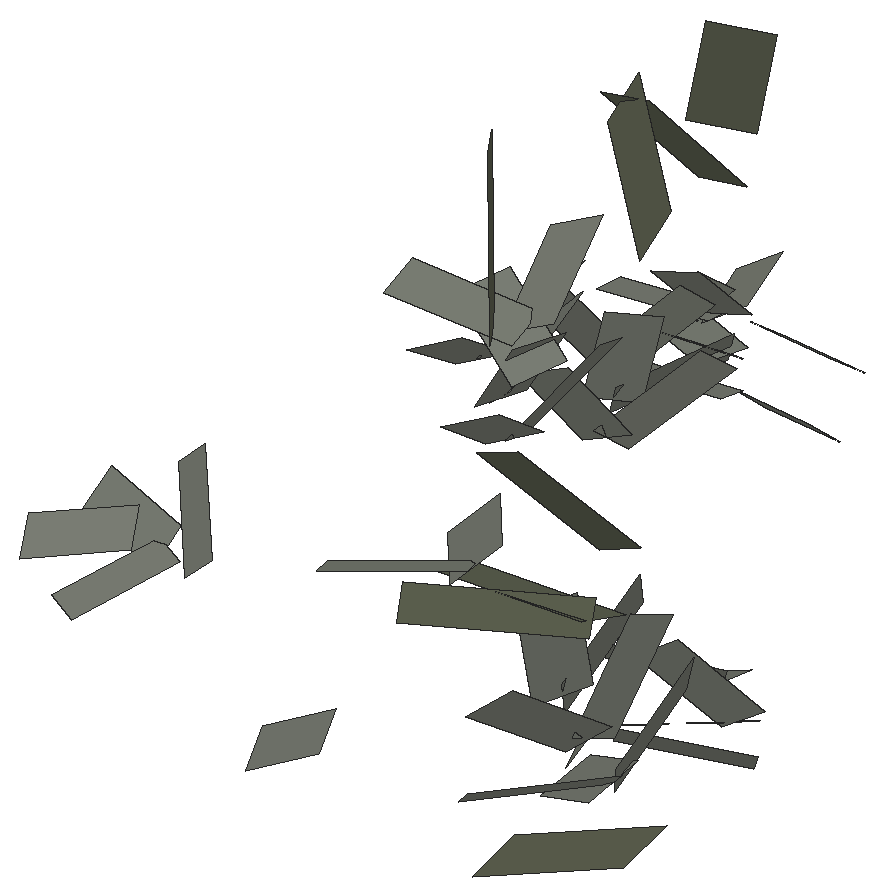
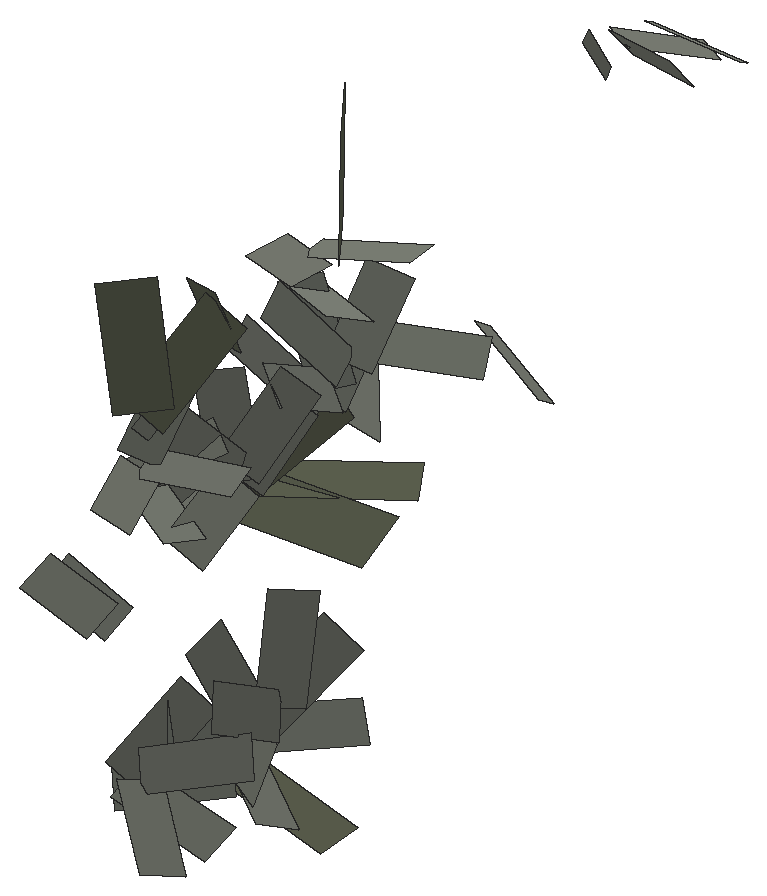
# SketchUp Ruby script. Lengths in inches.
U = 1.inch
M = Sketchup.active_model
def pt(a) = Geom::Point3d.new(a.map { |v| v * U })
def face(e, loops, mat)
  f = e.add_face(loops[0].map { |a| pt(a) })
  loops[1..].each { |l| e.add_face(l.map { |a| pt(a) }).erase! }
  f.material = f.back_material = mat if mat
  f
end
# faces: each face lists its corners as indices into pts; further lists are holes
def faces(e, pts, list, mat = nil) = list.each { |f| face(e, (f[0].is_a?(Array) ? f : [f]).map { |l| l.map { |i| pts[i] } }, mat) }
# xy, xz, yz: faces in a plane at the given z, y or x. An outline is a flat list of corners, or four numbers for a rectangle; further outlines are holes
def ring(l) = l.size == 4 ? [[l[0], l[1]], [l[2], l[1]], [l[2], l[3]], [l[0], l[3]]] : l.each_slice(2).to_a
def flat(e, list, mat, &to3) = list.each { |f| face(e, (f[0].is_a?(Array) ? f : [f]).map { |l| ring(l).map { |u, v| to3.(u, v) } }, mat) }
def xy(e, z, list, mat = nil) = flat(e, list, mat) { |x, y| [x, y, z] }
def xz(e, y, list, mat = nil) = flat(e, list, mat) { |x, z| [x, y, z] }
def yz(e, x, list, mat = nil) = flat(e, list, mat) { |y, z| [x, y, z] }
def lines(e, pts, list) = list.each { |a, b| e.add_line(pt(pts[a]), pt(pts[b])) }
# prism: a flat outline (further loops are holes) pulled along v
def prism(e, loops, v, mat = nil)
  f = face(e, loops, mat); d = Geom::Vector3d.new(v.map { |x| x * U })
  f.pushpull(f.normal.samedirection?(d) ? d.length : -d.length)
end
def box(e, o, s, mat = nil) = prism(e, [[o, [o[0] + s[0], o[1], o[2]], [o[0] + s[0], o[1] + s[1], o[2]], [o[0], o[1] + s[1], o[2]]]], [0, 0, s[2]], mat)
def at(x, y, z, deg = 0) = Geom::Transformation.translation(pt([x, y, z])) * Geom::Transformation.rotation(ORIGIN, Z_AXIS, deg.degrees)
def axes(o, x, y, z) = Geom::Transformation.new([*x, 0, *y, 0, *z, 0, *pt(o).to_a, 1])
def part(name) = M.definitions.add(name)
# library, detail: a bought-in or finely detailed component or shape, given as its bounding box
def library(name, o, s) = part(name).tap { |d| box(d.entities, o, s) }
def detail(e, o, s) = box(e.add_group.entities, o, s)
def put(e, d, t, mat = nil) = e.add_instance(d, t).tap { |i| i.material = mat if mat }
def group(e, t, mat = nil) = e.add_group.tap { |g| g.transformation = t; g.material = mat if mat }.entities
root = M.entities
M.materials.add("viburnumblaasdfas0df1w06d").color = [98, 102, 84]
M.materials.add("viburnumbladsadfasdfad0w122").color = [125, 129, 119]
c1 = part("Component\#315")
p = [[0.25,0,0],[2.05,0.01,0.35],[1.81,4.2,1.66],[0,4.19,1.3125]]
faces(c1.entities,p,[[0,1,2,3]],"viburnumbladsadfasdfad0w122")
c2 = part("viburnumblad2")
put(c2.entities,c1,axes([-19.23,-4.49,-32.18],[83.35428,0,0],[0,79.38502,0],[0,0,83.35428]))
c3 = part("Component\#314")
p = [[0.14,0,0],[2.58,0.05,0.25],[2.44,5.11,2.64],[0,5.05,2.39]]
faces(c3.entities,p,[[0,1,2,3]],"viburnumblaasdfas0df1w06d")
c4 = part("viburnumblad1\#2")
put(c4.entities,c3,axes([-37.25,6.23,19.31],[75.98784,0,0],[0,65.50676,0],[0,0,75.98784]))
put(root,c2,axes([1214.37,211.57,23.62],[-0.01,-0.00241,-0.00568],[-0.00201,-0.00892,0.00667],[-0.00557,0.00722,0.00577]))
put(root,c2,axes([1212.65,211.44,22.4375],[0.01,0.00241,0.00568],[0.00061,0.01041,-0.00507],[-0.00589,0.00485,0.00722]))
put(root,c4,axes([1215.02,215.93,27.11],[-0.01098,0.00138,-0.00403],[-0.00375,-0.01153,0.00597],[-0.00261,0.00614,0.00861]))
put(root,c2,axes([1213.71,206.3,25.72],[-0.00896,-0.00518,-0.00557],[0.00365,-0.01051,0.00351],[-0.00651,0.0014,0.00804]))
put(root,c2,axes([1212.83,206.35,23.64],[0.00946,-0.00383,0.00571],[0.00246,0.01108,0.00318],[-0.00637,-0.00125,0.00808]))
put(root,c2,axes([1213.04,209.58,11.62],[0.00591,-0.00596,0.00904],[0.00359,0.01104,0.00474],[-0.01042,0.00047,0.00632]))
put(root,c2,axes([1215.66,213.47,24.35],[-0.00169,0.00975,-0.0041],[-0.01002,-0.00286,-0.00259],[-0.00334,0.00343,0.00858]))
put(root,c2,axes([1214.08,208.34,10.625],[0.0076,0.00349,0.00917],[-0.0018,0.01107,-0.00252],[-0.00973,0.00035,0.00724]))
put(root,c4,axes([1213.88,217.59,27.8],[-0.00937,-0.00701,0.00111],[0.00657,-0.00694,0.00934],[-0.00422,0.00731,0.00713]))
put(root,c2,axes([1212.6,207.02,25.05],[0.00442,-0.0106,0.0025],[0.00816,0.00515,0.00656],[-0.00707,-0.00052,0.00766]))
put(root,c2,axes([1216.23,203.26,28.22],[-0.00228,0.01232,-0.00076],[-0.01222,-0.00233,-0.0015],[-0.0013,0.00061,0.01189]))
put(root,c2,axes([1214,209.75,12.84],[-0.00484,-0.0109,-0.00393],[0.00466,-0.0057,0.0098],[-0.01055,0.00253,0.0057]))
put(root,c2,axes([1215.96,184.97,28.88],[-0.00345,0.00905,0.004],[-0.00908,-0.00113,-0.00507],[-0.00385,-0.00506,0.00725]))
put(root,c4,axes([1215.91,210.54,27.46],[0.00699,0.00088,0.01038],[-0.00621,0.01278,0.0031],[-0.00893,-0.00592,0.00652]))
put(root,c2,axes([1216.04,213.85,12.28],[-0.00463,0.00496,-0.0092],[-0.00796,-0.0082,-0.00042],[-0.00678,0.00624,0.00678]))
put(root,c2,axes([1215.39,207.8,10.1],[0.00505,0.01138,0.0041],[-0.00637,0.00552,-0.00732],[-0.00911,0.00107,0.00791]))
put(root,c2,axes([1215.05,213.72,11.24],[0.00707,0.00889,0.00124],[-0.00553,0.00556,-0.00832],[-0.00707,0.00455,0.00775]))
put(root,c2,axes([1215.39,208.92,12.27],[-0.0076,-0.00349,-0.00917],[-0.00045,-0.01161,0.00442],[-0.00992,0.00325,0.00636]))
put(root,c2,axes([1215.64,209.89,22.02],[-0.01044,-0.00252,-0.00593],[-0.00181,-0.00803,0.006],[-0.00557,0.00722,0.00577]))
put(root,c2,axes([1215.6,213.1,22.99],[0.00555,0.00919,-0.00035],[-0.00852,0.00498,-0.00446],[-0.00353,0.00247,0.00881]))
put(root,c2,axes([1216.02,203.52,26.65],[0.00658,0.00998,0.00148],[-0.01117,0.00758,-0.00127],[-0.00153,-0.00054,0.01185]))
put(root,c2,axes([1216.4,208.11,11.28],[-0.00567,0.00572,-0.00867],[-0.00649,-0.01145,-0.00331],[-0.00924,0.00313,0.00728]))
put(root,c2,axes([1216.08,185.87,27.89],[0.0036,0.00676,0.00701],[-0.00902,0.00536,-0.00055],[-0.00386,-0.00586,0.0067]))
put(root,c2,axes([1215.15,206.05,23.6],[-0.00935,-0.0054,-0.00582],[0.00328,-0.00946,0.00316],[-0.00651,0.0014,0.00804]))
put(root,c2,axes([1213.89,206.83,24.28],[-0.00321,-0.01115,-0.00217],[0.00909,-0.00398,0.00703],[-0.00713,0.00058,0.00765]))
put(root,c2,axes([1216.59,213.01,11.04],[0.00173,0.0098,-0.00563],[-0.00961,-0.00223,-0.00684],[-0.00663,0.00549,0.00752]))
put(root,c2,axes([1214.79,214.24,23.66],[0.00954,0.00326,0.00362],[-0.00223,0.01005,-0.00307],[-0.00429,0.00184,0.00864]))
put(root,c2,axes([1213.78,212.4,22.59],[-0.00132,-0.00974,0.00592],[0.00922,0.00313,0.00644],[-0.00695,0.00574,0.0058]))
put(root,c2,axes([1216.81,212.68,22.44],[-0.00122,0.00857,-0.00461],[-0.01002,-0.00286,-0.00259],[-0.0035,0.00446,0.00809]))
put(root,c4,axes([1218.18,207.02,8.81],[-0.00086,0.01375,0.00031],[-0.0113,-0.00049,-0.01107],[-0.00962,-0.00074,0.00907]))
put(root,c2,axes([1214.87,211.36,22.1875],[-0.008,-0.00859,0.00017],[0.00566,-0.00462,0.00938],[-0.00647,0.00667,0.0055]))
put(root,c2,axes([1213.74,211.2,21.5],[0.00614,-0.00518,0.0082],[0.00724,0.00927,0.00063],[-0.0067,0.00499,0.00652]))
put(root,c4,axes([1218.35,204.58,18.19],[-0.00055,0.01258,-0.0057],[-0.01484,-0.00329,-0.00573],[-0.0051,0.00524,0.0099]))
put(root,c4,axes([1215.28,204.09,27.6],[0.0095,-0.01111,0.00288],[0.00361,0.00703,0.01484],[-0.01096,-0.00785,0.00554]))
put(root,c2,axes([1216.89,217.94,21.52],[0.00286,0.007,-0.00749],[-0.01015,0.00031,-0.00351],[-0.0019,0.00782,0.00576]))
put(root,c2,axes([1216.96,213.55,23.48],[-0.00794,0.00459,-0.00546],[-0.00557,-0.00804,0.00123],[-0.00382,0.00415,0.0081]))
put(root,c2,axes([1217.56,199.25,22.7],[-0.00445,0.01048,-0.00645],[-0.00976,-0.00718,-0.00494],[-0.00749,0.00313,0.01026]))
put(root,c2,axes([1215.16,204.15,27.92],[0.01197,0.00238,0.00293],[-0.00273,0.01289,0.0007],[-0.00248,-0.00118,0.01162]))
put(root,c2,axes([1214.73,209.89,11.2],[0.00076,-0.01192,0.00361],[0.0064,0.00373,0.01004],[-0.01075,0.00137,0.00569]))
put(root,c2,axes([1214,206.65,22.875],[0.00424,-0.01017,0.0024],[0.00881,0.00556,0.00708],[-0.00707,-0.00052,0.00766]))
put(root,c4,axes([1218.84,204.2,18.17],[-0.00719,0.01195,-0.00129],[-0.01278,-0.0083,-0.00564],[-0.00429,-0.00131,0.01125]))
put(root,c2,axes([1217.24,185.76,28.57],[-0.00848,0.00604,-0.00136],[-0.00422,-0.00741,-0.00622],[-0.00446,-0.0043,0.00739]))
put(root,c2,axes([1216.46,199.79,21.59],[0.00877,0.00751,0.00615],[-0.00546,0.01067,-0.00523],[-0.00802,0.00094,0.01029]))
put(root,c2,axes([1216.52,214.52,24.43],[-0.00954,-0.00326,-0.00362],[0.00113,-0.0093,0.00507],[-0.00471,0.00422,0.00764]))
put(root,c2,axes([1217.42,192.15,19.2],[-0.00095,0.00927,0.00479],[-0.00714,0.003,-0.00705],[-0.00723,-0.00378,0.00515]))
put(root,c2,axes([1215.33,209.14,9.88],[0.00644,-0.0055,0.00764],[0.00359,0.01104,0.00474],[-0.00972,-0.00018,0.00726]))
put(root,c4,axes([1218.28,206.83,19.68],[-0.01073,0.0028,-0.00658],[-0.00691,-0.01149,0.00571],[-0.00344,0.00773,0.00806]))
put(root,c2,axes([1218.03,212.86,10.44],[-0.00445,0.00477,-0.00883],[-0.0086,-0.00885,-0.00045],[-0.00678,0.00624,0.00678]))
put(root,c2,axes([1216.47,186.96,27.25],[0.00821,0.00049,0.00568],[-0.00435,0.00902,0.00515],[-0.00448,-0.00623,0.00604]))
put(root,c2,axes([1217.66,216.02,20.34],[0.0028,0.00563,-0.00742],[-0.01015,0.00031,-0.00351],[-0.00158,0.00853,0.00492]))
put(root,c2,axes([1217.41,213.98,11.28],[-0.00828,-0.00278,-0.00738],[-0.00265,-0.00909,0.0064],[-0.00743,0.00635,0.00594]))
put(root,c2,axes([1214.97,210.62,20.95],[-0.00127,-0.00935,0.00568],[0.00996,0.00338,0.00695],[-0.00695,0.00574,0.0058]))
